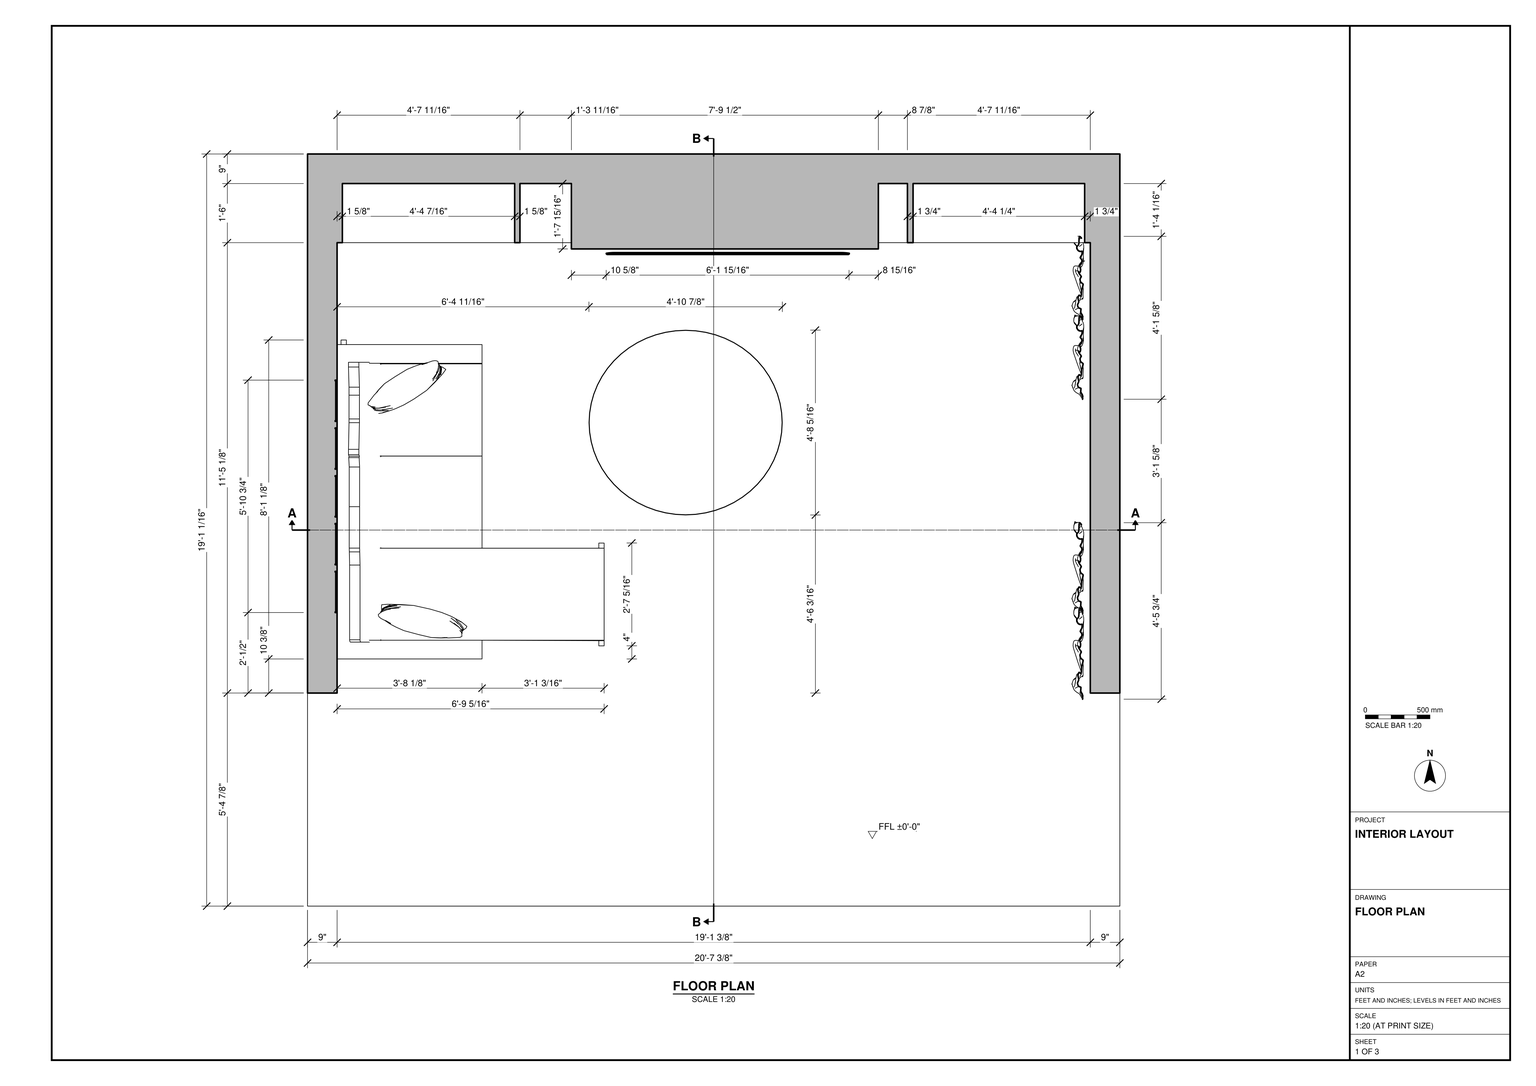
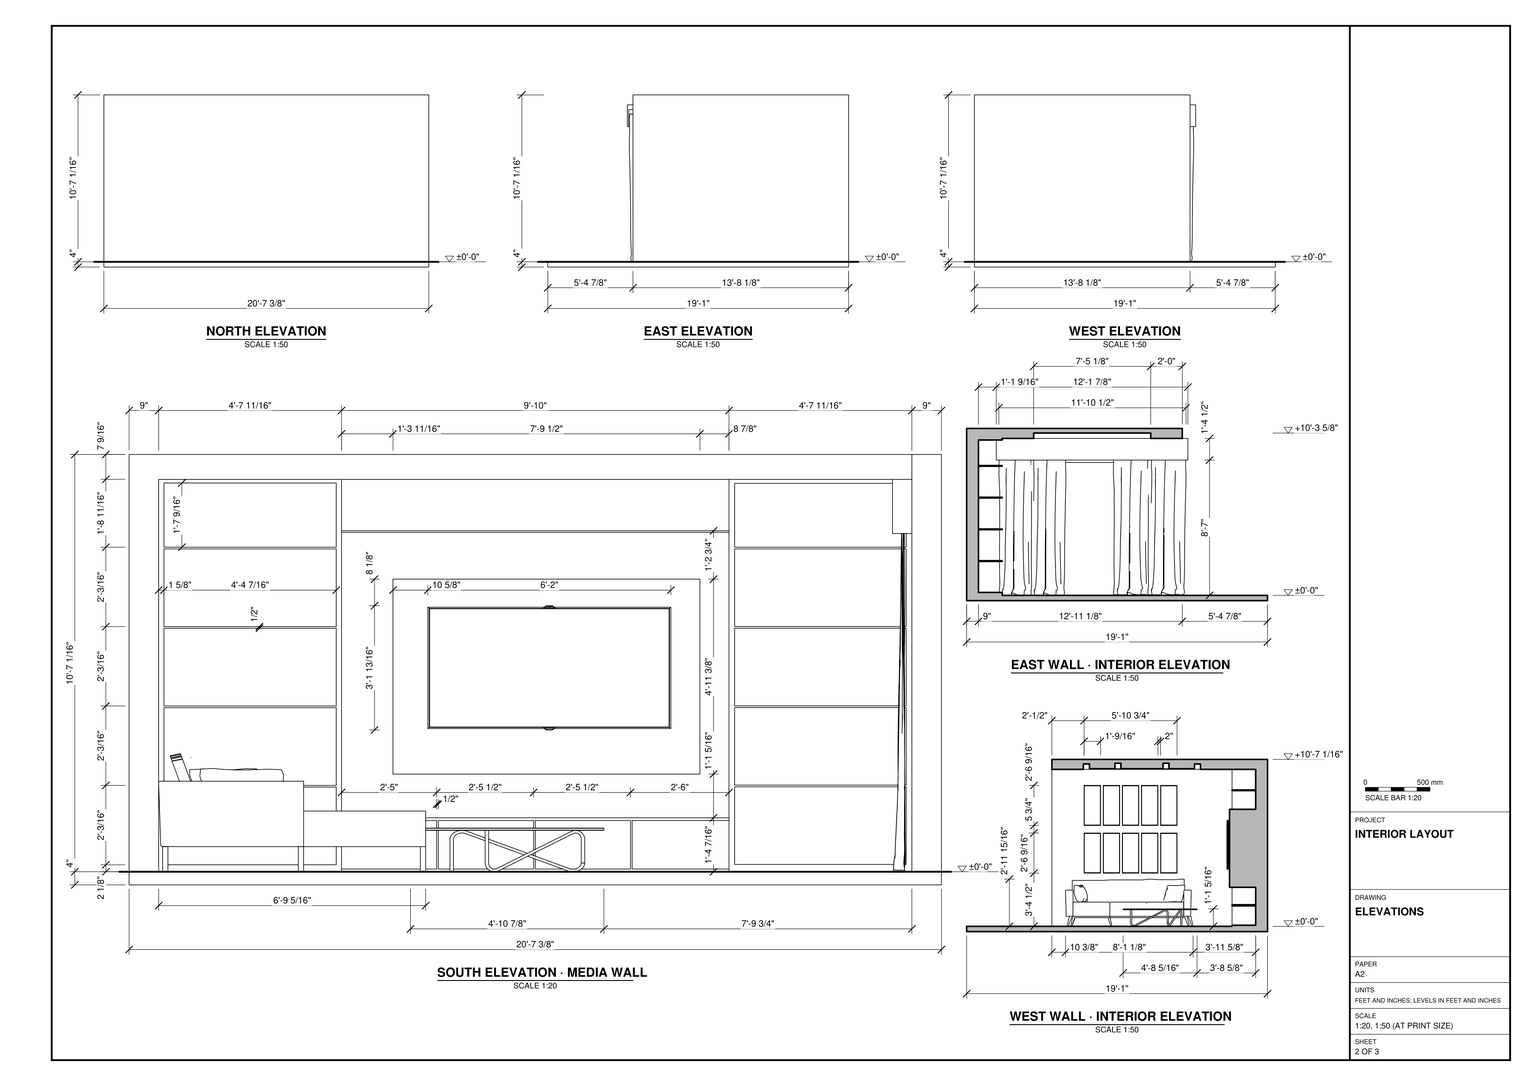
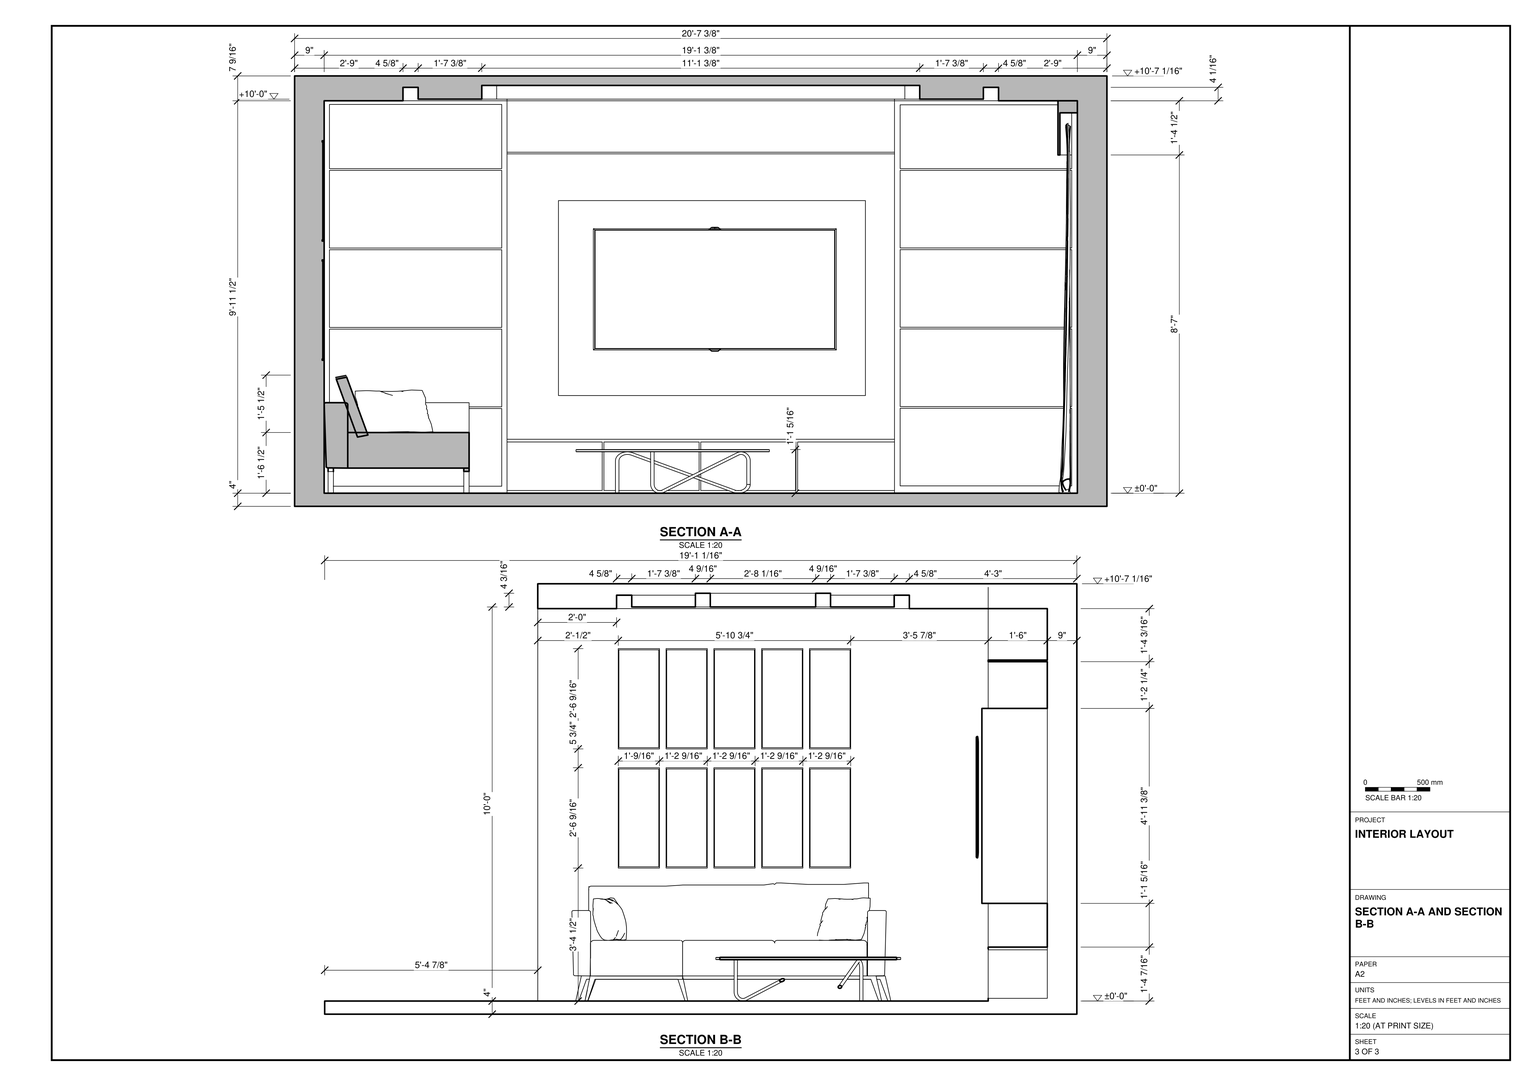
Build the living room in SketchUp from task_files/diagram_01.pdf. Work in feet and inches. Set the finished floor at ±0'-0" and use overall dimensions of 20'-7 3/8" wide, 19'-1 1/16" deep and 10'-11 1/16" high. Model the 4" floor slab, the 9" rear and side walls, and the ceiling over the seating area. Leave the front open, with the floor extending 5'-4 7/8" beyond the ends of the side walls. Use the sections to set out the recesses in the underside of the ceiling.

Build the media wall across the rear of the room. Use the elevation to lay out the tall shelving bays on either side, the projecting central panel with the television, and the low divided unit beneath it. Place the corner sofa along the west wall with its return towards the centre of the room at the open end. Size the sofa and low coffee table from their plan footprints, and use the sections for their profiles. Place the wall pictures above the sofa and the curtained window area on the opposite wall as shown.

Decor and loose items may be any suitable library components. Keep shell elements and individual furniture and joinery pieces in separate groups or components, and use components for repeated parts. Save one SketchUp model as output_files/living_room_with_a_built_in_media_wall.skp.

# SketchUp Ruby script. Lengths in inches.
U = 1.inch
M = Sketchup.active_model
def pt(a) = Geom::Point3d.new(a.map { |v| v * U })
def face(e, loops, mat)
  f = e.add_face(loops[0].map { |a| pt(a) })
  loops[1..].each { |l| e.add_face(l.map { |a| pt(a) }).erase! }
  f.material = f.back_material = mat if mat
  f
end
# faces: each face lists its corners as indices into pts; further lists are holes
def faces(e, pts, list, mat = nil) = list.each { |f| face(e, (f[0].is_a?(Array) ? f : [f]).map { |l| l.map { |i| pts[i] } }, mat) }
# xy, xz, yz: faces in a plane at the given z, y or x. An outline is a flat list of corners, or four numbers for a rectangle; further outlines are holes
def ring(l) = l.size == 4 ? [[l[0], l[1]], [l[2], l[1]], [l[2], l[3]], [l[0], l[3]]] : l.each_slice(2).to_a
def flat(e, list, mat, &to3) = list.each { |f| face(e, (f[0].is_a?(Array) ? f : [f]).map { |l| ring(l).map { |u, v| to3.(u, v) } }, mat) }
def xy(e, z, list, mat = nil) = flat(e, list, mat) { |x, y| [x, y, z] }
def xz(e, y, list, mat = nil) = flat(e, list, mat) { |x, z| [x, y, z] }
def yz(e, x, list, mat = nil) = flat(e, list, mat) { |y, z| [x, y, z] }
def lines(e, pts, list) = list.each { |a, b| e.add_line(pt(pts[a]), pt(pts[b])) }
# prism: a flat outline (further loops are holes) pulled along v
def prism(e, loops, v, mat = nil)
  f = face(e, loops, mat); d = Geom::Vector3d.new(v.map { |x| x * U })
  f.pushpull(f.normal.samedirection?(d) ? d.length : -d.length)
end
def box(e, o, s, mat = nil) = prism(e, [[o, [o[0] + s[0], o[1], o[2]], [o[0] + s[0], o[1] + s[1], o[2]], [o[0], o[1] + s[1], o[2]]]], [0, 0, s[2]], mat)
def at(x, y, z, deg = 0) = Geom::Transformation.translation(pt([x, y, z])) * Geom::Transformation.rotation(ORIGIN, Z_AXIS, deg.degrees)
def axes(o, x, y, z) = Geom::Transformation.new([*x, 0, *y, 0, *z, 0, *pt(o).to_a, 1])
def part(name) = M.definitions.add(name)
# library, detail: a bought-in or finely detailed component or shape, given as its bounding box
def library(name, o, s) = part(name).tap { |d| box(d.entities, o, s) }
def detail(e, o, s) = box(e.add_group.entities, o, s)
def put(e, d, t, mat = nil) = e.add_instance(d, t).tap { |i| i.material = mat if mat }
def group(e, t, mat = nil) = e.add_group.tap { |g| g.transformation = t; g.material = mat if mat }.entities
root = M.entities
M.materials.add("Emissive").color = [255, 255, 255]
M.materials.add("Marble_01_1K").color = [230, 221, 211]
M.materials.add("Marble_03_1K").color = [175, 182, 201]
M.materials.add("Marble_06_1K").color = [165, 150, 147]
M.materials.add("Wood_Floor_01_1K").color = [146, 111, 76]
M.materials.add("Wood_Floor_12_1K").color = [92, 75, 65]
M.materials.add("Wood_Planks_01_1K").color = [69, 67, 63]
M.materials.add("Wood_Veneer_15_1K").color = [103, 69, 45]
M.materials.add("[Color_008]").color = [30, 30, 30]
c1 = library("sofa+black+corner",[1.125,-27.17,-0.04],[86.72,59.42,36.47])
c2 = library("coffee+table",[-23.75,-21.65,0],[45.4,45.4,13.31])
c3 = library("Window curtains",[0,0,0],[5.91,79.92,51.3])
c4 = part("Rectangular panel")
xy(c4.entities,0,[[[0,0,24.61,31.5],[0.39,0.39,24.21,31.1]]],"[Color_008]")
xy(c4.entities,0.2,[[0.39,0.39,24.21,31.1]],"[Color_008]")
xy(c4.entities,0.59,[[[0,0,24.61,31.5],[0.39,0.39,24.21,31.1]]],"[Color_008]")
xz(c4.entities,0,[[0,0,24.61,0.59]],"[Color_008]")
xz(c4.entities,0.39,[[0.39,0.2,24.21,0.59]],"[Color_008]")
xz(c4.entities,31.1,[[0.39,0.2,24.21,0.59]],"[Color_008]")
xz(c4.entities,31.5,[[0,0,24.61,0.59]],"[Color_008]")
yz(c4.entities,0,[[0,0,31.5,0.59]],"[Color_008]")
yz(c4.entities,0.39,[[0.39,0.2,31.1,0.59]],"[Color_008]")
yz(c4.entities,24.21,[[0.39,0.2,31.1,0.59]],"[Color_008]")
yz(c4.entities,24.61,[[0,0,31.5,0.59]],"[Color_008]")
c5 = part("black+and+white+pictures")
g1 = group(c5.entities,at(0,0.875,14.87))
g2 = group(g1,at(0,0,0))
put(g2,c4,axes([0,0,0],[1,0,0],[0,0,1],[0,-1,0]))
g3 = group(g1,at(57.09,0,37.4))
put(g3,c4,axes([0,0,0],[1,0,0],[0,0,1],[0,-1,0]))
g4 = group(g1,at(28.54,0,37.4))
put(g4,c4,axes([0,0,0],[1,0,0],[0,0,1],[0,-1,0]))
g5 = group(g1,at(0,0,37.4))
put(g5,c4,axes([0,0,0],[1,0,0],[0,0,1],[0,-1,0]))
g6 = group(g1,at(114.17,0,0))
put(g6,c4,axes([0,0,0],[1,0,0],[0,0,1],[0,-1,0]))
g7 = group(g1,at(85.63,0,0))
put(g7,c4,axes([0,0,0],[1,0,0],[0,0,1],[0,-1,0]))
g8 = group(g1,at(57.09,0,0))
put(g8,c4,axes([0,0,0],[1,0,0],[0,0,1],[0,-1,0]))
g9 = group(g1,at(28.54,0,0))
put(g9,c4,axes([0,0,0],[1,0,0],[0,0,1],[0,-1,0]))
g10 = group(g1,at(114.17,0,37.4))
put(g10,c4,axes([0,0,0],[1,0,0],[0,0,1],[0,-1,0]))
g11 = group(g1,at(85.63,0,37.4))
put(g11,c4,axes([0,0,0],[1,0,0],[0,0,1],[0,-1,0]))
c6 = library("download?mid=50c7180b9fccec56d493bfe20f94b6ab&ctyp=sp&cv=p8.",[149.43,43.83,17.86],[74.75,0.57,42.04])
c7 = library("Spot Light",[-5.1,-5.1,-11.05],[10.2,10.2,11.05])
c8 = library("Rectangle Light",[-3.26,-3.26,-3.26],[6.52,6.52,3.26])
xy(root,0,[[0,0,247.35,229.04]])
xy(root,4,[[0,0,247.35,0,247.35,64.89,238.35,64.89,238.35,202.04,9,202.04,9,64.89,0,64.89]],"Marble_03_1K")
xy(root,4.82,[[64.68,202.04,65.51,220.04],[65.51,202.04,93.67,220.04],[94.18,202.04,123.18,220.04],[123.68,202.04,152.67,220.04],[153.17,202.04,182.67,220.04]],"Wood_Veneer_15_1K")
xy(root,6.125,[[10.61,202.04,63.07,220.04]],"Wood_Floor_01_1K")
xy(root,6.24,[[184.39,202.04,236.63,220.04]],"Wood_Veneer_15_1K")
xy(root,19.6,[[64.68,202.04,65.51,220.04],[65.51,202.04,93.67,220.04],[94.18,202.04,123.18,220.04],[123.68,202.04,152.67,220.04],[153.17,202.04,182.67,220.04]],"Wood_Veneer_15_1K")
xy(root,20.42,[[64.68,202.04,182.67,220.04]],"Wood_Floor_01_1K")
xy(root,29.79,[[10.61,202.04,63.07,220.04]],"Wood_Floor_01_1K")
xy(root,29.87,[[184.39,202.04,236.63,220.04]],"Wood_Veneer_15_1K")
xy(root,30.3,[[10.61,202.04,63.07,220.04]],"Wood_Floor_01_1K")
xy(root,30.39,[[184.39,202.04,236.63,220.04]],"Wood_Floor_01_1K")
xy(root,33.74,[[80.34,200.125,173.82,220.04]],"Marble_06_1K")
xy(root,53.96,[[10.61,202.04,63.07,220.04]],"Wood_Floor_01_1K")
xy(root,54.02,[[184.39,202.04,236.63,220.04]],"Wood_Veneer_15_1K")
xy(root,54.48,[[10.61,202.04,63.07,220.04]],"Wood_Floor_01_1K")
xy(root,54.54,[[184.39,202.04,236.63,220.04]],"Wood_Floor_01_1K")
xy(root,78.14,[[10.61,202.04,63.07,220.04]],"Wood_Floor_01_1K")
xy(root,78.17,[[184.39,202.04,236.63,220.04]],"Wood_Veneer_15_1K")
xy(root,78.66,[[10.61,202.04,63.07,220.04]],"Wood_Floor_01_1K")
xy(root,78.69,[[184.39,202.04,236.63,220.04]],"Wood_Floor_01_1K")
xy(root,93.11,[[80.34,200.125,173.82,220.04]],"Marble_06_1K")
xy(root,102.32,[[10.61,202.04,63.07,220.04]],"Wood_Floor_01_1K")
xy(root,102.32,[[184.39,202.04,236.63,220.04]],"Wood_Veneer_15_1K")
xy(root,102.83,[[184.39,202.04,236.63,220.04]])
xy(root,102.83,[[10.61,202.04,63.07,220.04]],"Wood_Floor_01_1K")
xy(root,107.34,[[64.68,202.04,182.67,220.04]],"Wood_Floor_01_1K")
xy(root,107.83,[[64.68,202.04,65.18,220.04]])
xy(root,107.83,[[65.18,202.04,182.67,220.04]],"Wood_Floor_01_1K")
xy(root,122.28,[[184.39,202.04,236.63,220.04]],"Wood_Veneer_15_1K")
xy(root,122.39,[[10.61,202.04,63.07,220.04]],"Wood_Floor_01_1K")
xy(root,123.51,[[[9,64.89,238.35,202.04],[33,88.89,214.35,178.04]],[64.68,202.04,65.18,220.04]])
xy(root,123.51,[[65.18,202.04,182.67,220.04]],"Wood_Floor_01_1K")
xy(root,124,[[[37.62,93.5,209.73,173.42],[57,112.89,190.35,154.04]],[61.53,117.42,185.82,149.51]])
xy(root,127.59,[[[33,88.89,214.35,178.04],[37.62,93.5,209.73,173.42]]],"Emissive")
xy(root,128.18,[[[57,112.89,190.35,154.04],[61.53,117.42,185.82,149.51]]],"Emissive")
xy(root,131.07,[[0,64.89,247.35,229.04]])
xz(root,0,[[0,0,247.35,4]])
xz(root,64.89,[[0,4,9,4,9,123.51,238.35,123.51,238.35,131.07,0,131.07],[238.35,4,247.35,131.07]])
xz(root,88.89,[[33,123.51,214.35,127.59]],"Emissive")
xz(root,93.5,[[37.62,124,209.73,127.59]],"Emissive")
xz(root,112.89,[[57,124,190.35,128.18]],"Emissive")
xz(root,117.42,[[61.53,124,185.82,128.18]])
xz(root,149.51,[[61.53,124,64.68,128.18],[64.68,124,182.67,128.18],[182.67,124,185.82,128.18]])
xz(root,154.04,[[182.67,124,190.35,128.18]])
xz(root,154.04,[[57,124,64.68,128.18],[64.68,124,182.67,128.18]],"Emissive")
xz(root,173.42,[[37.62,124,64.68,127.59],[64.68,124,182.67,127.59],[182.67,124,209.73,127.59]])
xz(root,178.04,[[64.68,123.51,182.67,127.59],[182.67,123.51,214.35,127.59]])
xz(root,178.04,[[33,123.51,64.68,127.59]],"Emissive")
xz(root,200.125,[[80.34,33.74,173.82,93.11]],"Marble_06_1K")
xz(root,202.04,[[[9,4,64.68,123.51],[10.61,78.66,63.07,102.32],[10.61,6.125,63.07,29.79],[10.61,30.3,63.07,53.96],[10.61,54.48,63.07,78.14],[10.61,102.83,63.07,122.39]],[64.68,107.34,182.67,107.83]],"Wood_Planks_01_1K")
xz(root,202.04,[[[64.68,4,182.67,4,182.67,4.82,153.17,4.82,153.17,19.6,182.67,19.6,182.67,20.42,64.68,20.42,64.68,19.6,93.67,19.6,93.67,4.82,64.68,4.82],[94.18,4.82,123.18,19.6],[123.68,4.82,152.67,19.6]],[[182.67,4,238.35,123.51],[184.39,30.39,236.63,54.02],[184.39,6.24,236.63,29.87],[184.39,54.54,236.63,78.17],[184.39,78.69,236.63,102.32],[184.39,102.83,236.63,122.28]]],"Wood_Veneer_15_1K")
xz(root,220.04,[[64.68,4.82,93.67,19.6],[94.18,4.82,123.18,19.6],[123.68,4.82,152.67,19.6],[153.17,4.82,182.67,19.6],[10.61,6.125,63.07,29.79],
  [184.39,6.24,236.63,29.87],[[64.68,20.42,182.67,107.34],[80.34,33.74,173.82,93.11]],[10.61,30.3,63.07,53.96],[184.39,30.39,236.63,54.02],[10.61,54.48,63.07,78.14],
  [184.39,54.54,236.63,78.17],[10.61,78.66,63.07,102.32],[184.39,78.69,236.63,102.32],[10.61,102.83,63.07,122.39],[184.39,102.83,236.63,122.28],
  [64.68,107.83,182.67,123.51]],"Wood_Floor_12_1K")
xz(root,229.04,[[0,0,247.35,131.07]])
yz(root,0,[[0,0,0,4,64.89,4,64.89,131.07,229.04,131.07,229.04,0]])
yz(root,9,[[64.89,4,202.04,123.51]])
yz(root,10.61,[[202.04,6.125,220.04,29.79],[202.04,30.3,220.04,53.96],[202.04,54.48,220.04,78.14],[202.04,78.66,220.04,102.32],[202.04,102.83,220.04,122.39]],"Wood_Floor_01_1K")
yz(root,33,[[88.89,123.51,178.04,127.59]])
yz(root,37.62,[[93.5,124,173.42,127.59]])
yz(root,57,[[112.89,124,154.04,128.18]],"Emissive")
yz(root,61.53,[[117.42,124,149.51,128.18]],"Emissive")
yz(root,63.07,[[202.04,6.125,220.04,29.79],[202.04,30.3,220.04,53.96],[202.04,54.48,220.04,78.14],[202.04,78.66,220.04,102.32],[202.04,102.83,220.04,122.39]],"Wood_Floor_01_1K")
yz(root,64.68,[[202.04,20.42,220.04,107.34],[202.04,107.83,220.04,123.51]],"Wood_Floor_01_1K")
yz(root,64.68,[[202.04,4.82,220.04,19.6]],"Wood_Veneer_15_1K")
yz(root,80.34,[[200.125,33.74,220.04,93.11]],"Marble_06_1K")
yz(root,93.67,[[202.04,4.82,220.04,19.6]],"Wood_Veneer_15_1K")
yz(root,94.18,[[202.04,4.82,220.04,19.6]],"Wood_Veneer_15_1K")
yz(root,123.18,[[202.04,4.82,220.04,19.6]],"Wood_Veneer_15_1K")
yz(root,123.68,[[202.04,4.82,220.04,19.6]],"Wood_Veneer_15_1K")
yz(root,152.67,[[202.04,4.82,220.04,19.6]],"Wood_Veneer_15_1K")
yz(root,153.17,[[202.04,4.82,220.04,19.6]],"Wood_Veneer_15_1K")
yz(root,173.82,[[200.125,33.74,220.04,93.11]])
yz(root,182.67,[[202.04,107.83,220.04,123.51]],"Wood_Floor_01_1K")
yz(root,182.67,[[202.04,4.82,220.04,19.6],[202.04,20.42,220.04,107.34]],"Wood_Veneer_15_1K")
yz(root,184.39,[[202.04,6.24,220.04,29.87],[202.04,30.39,220.04,54.02],[202.04,54.54,220.04,78.17],[202.04,78.69,220.04,102.32],[202.04,102.83,220.04,122.28]],"Wood_Veneer_15_1K")
yz(root,185.82,[[117.42,124,149.51,128.18]])
yz(root,190.35,[[112.89,124,154.04,128.18]],"Emissive")
yz(root,209.73,[[93.5,124,173.42,127.59]],"Emissive")
yz(root,214.35,[[88.89,123.51,178.04,127.59]],"Emissive")
yz(root,236.63,[[202.04,6.24,220.04,29.87],[202.04,30.39,220.04,54.02],[202.04,54.54,220.04,78.17],[202.04,78.69,220.04,102.32],[202.04,102.83,220.04,122.28]],"Wood_Veneer_15_1K")
yz(root,238.35,[[64.89,4,202.04,105.16]])
yz(root,238.35,[[64.89,105.16,202.04,123.51]],"Marble_01_1K")
yz(root,247.35,[[0,0,229.04,0,229.04,131.07,64.89,131.07,64.89,4,0,4]])
p = [[238.35,202.04,123.51],[238.35,202.04,130],[182.67,202.04,123.51],[182.67,202.04,130],[9,202.04,123.51],[9,202.04,130],
  [64.68,202.04,123.51],[64.68,202.04,130]]
lines(root,p,[[0,1],[2,3],[4,5],[6,7]])
put(root,c1,axes([53.14,74.01,4.04],[0,1.12,0],[-1.36858,0,0],[0,0,1]))
put(root,c2,axes([115.13,147.25,4],[1.36,0,0],[0,1.3,0],[0,0,1]))
put(root,c3,axes([232.45,60.61,4],[1,0,0],[0,1.8252,0],[0,0,2.32936]))
put(root,c5,axes([9.29,160.17,30.07],[0,-0.51,0],[-1,0,0],[0,0,0.97]))
put(root,c6,axes([-56.97,154.6,31.11],[0.99,0,0],[0,1,0],[0,0,0.9]))
put(root,c7,at(9,111.02,123.51))
put(root,c8,axes([34.03,75.77,123.5],[-1,0,0],[0,1,0],[0,0,1]))
